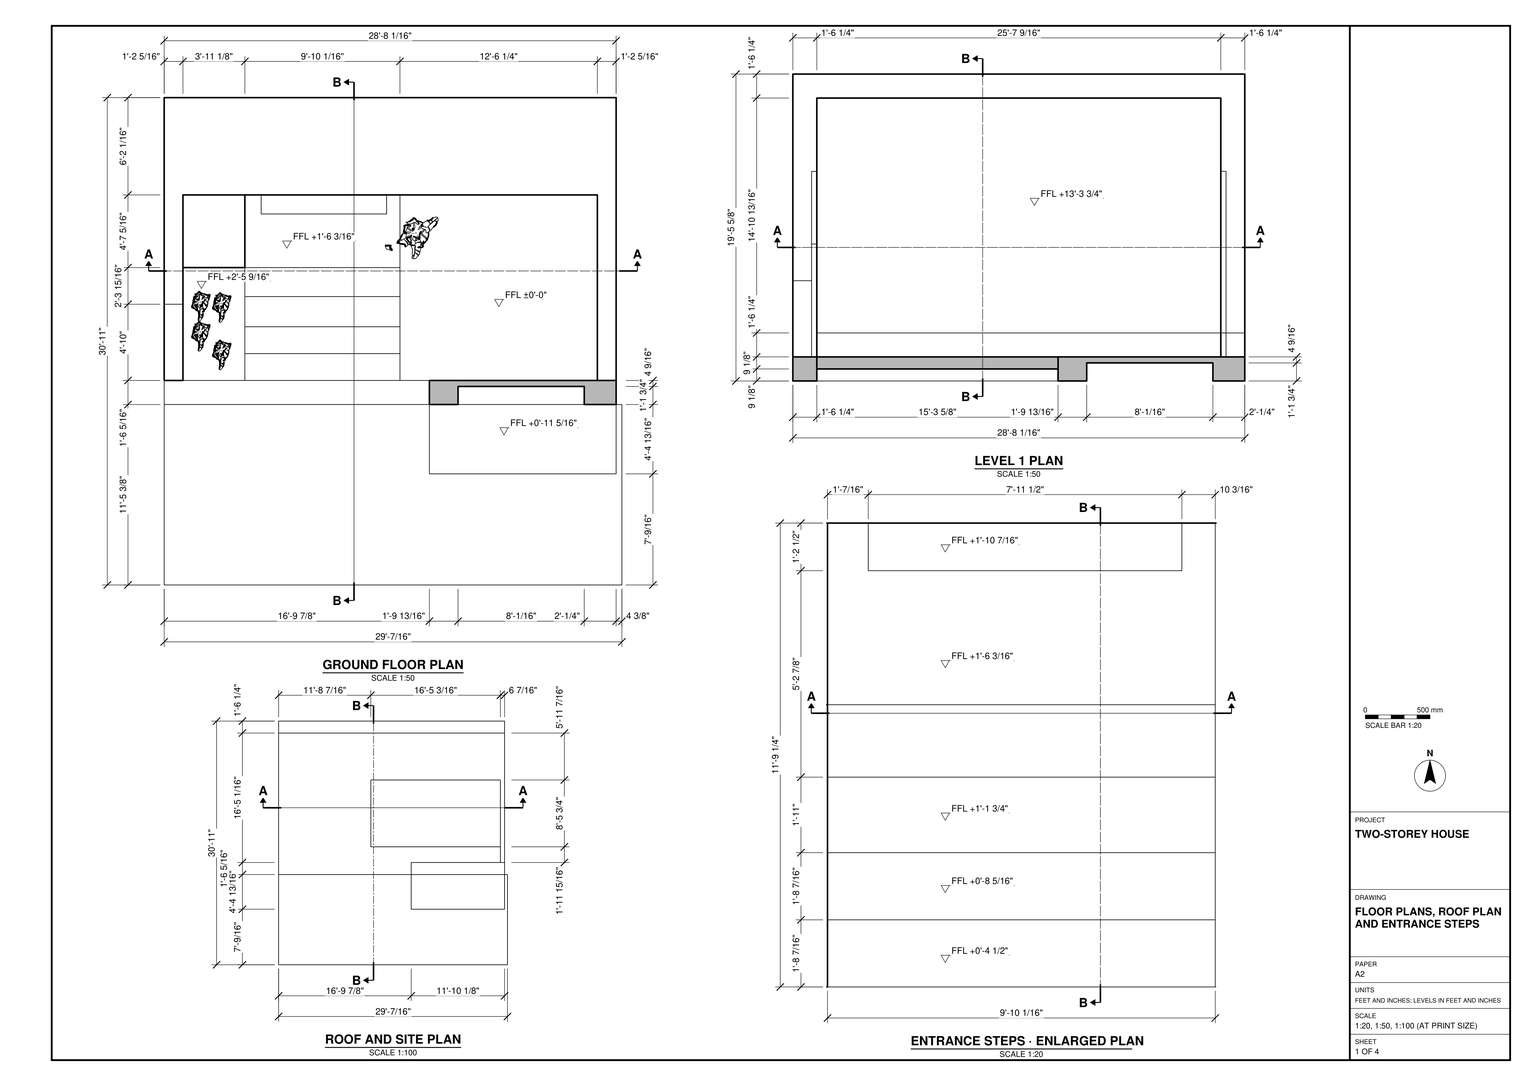
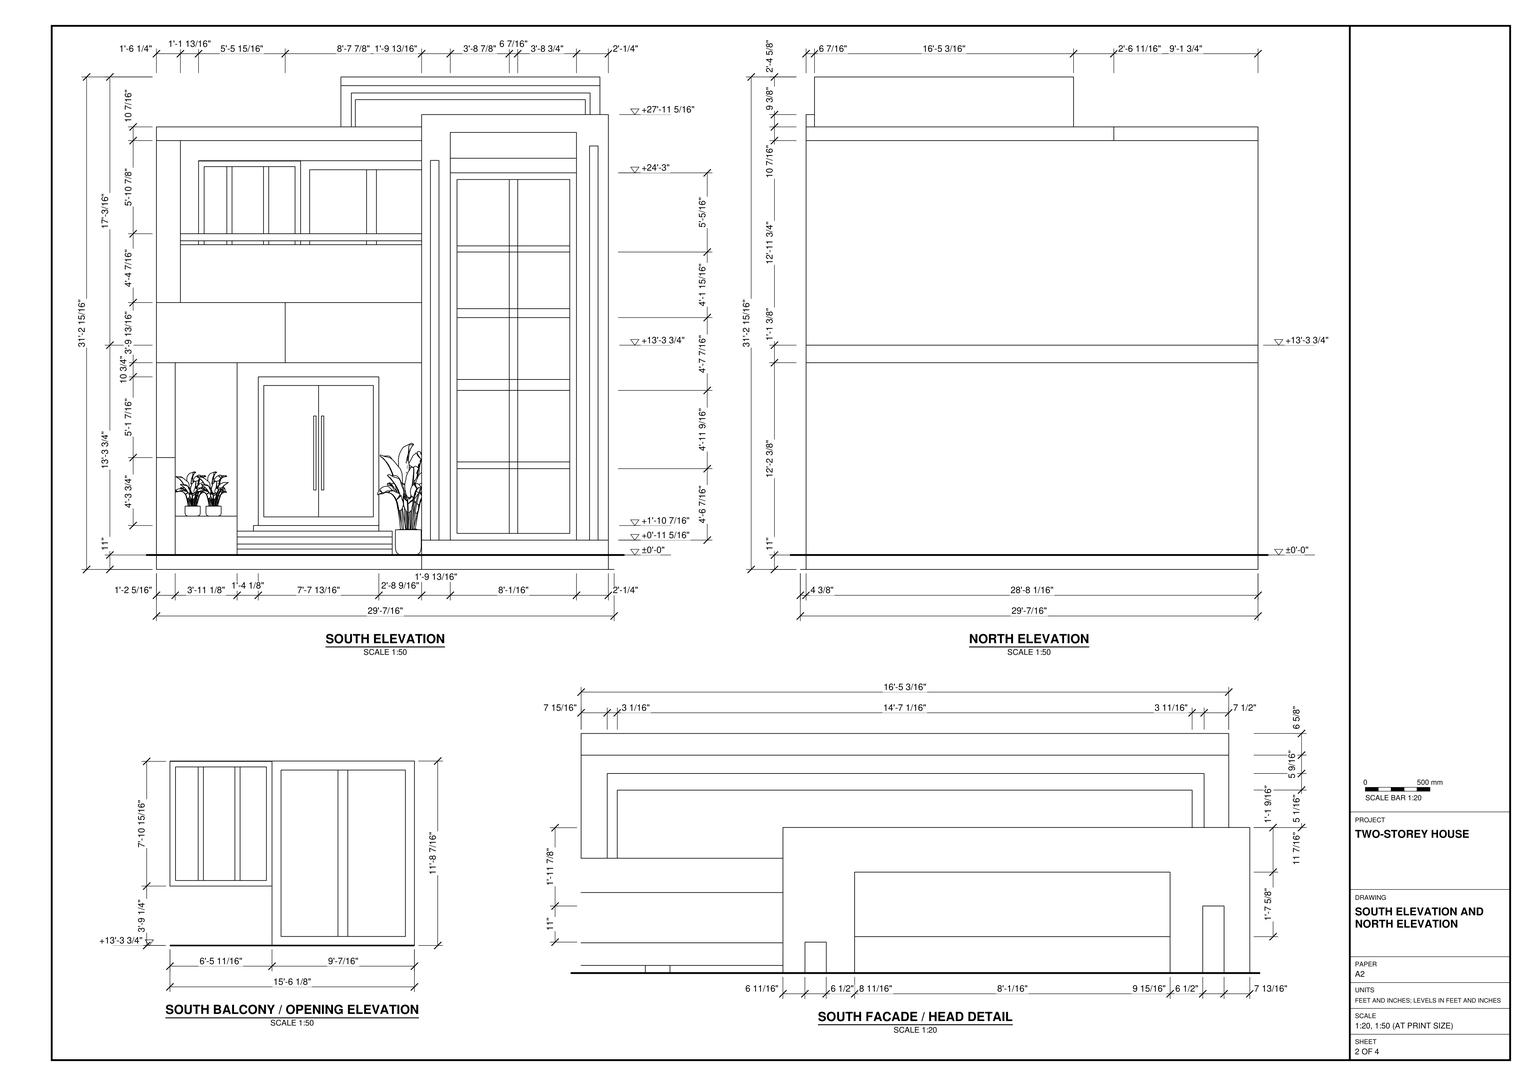
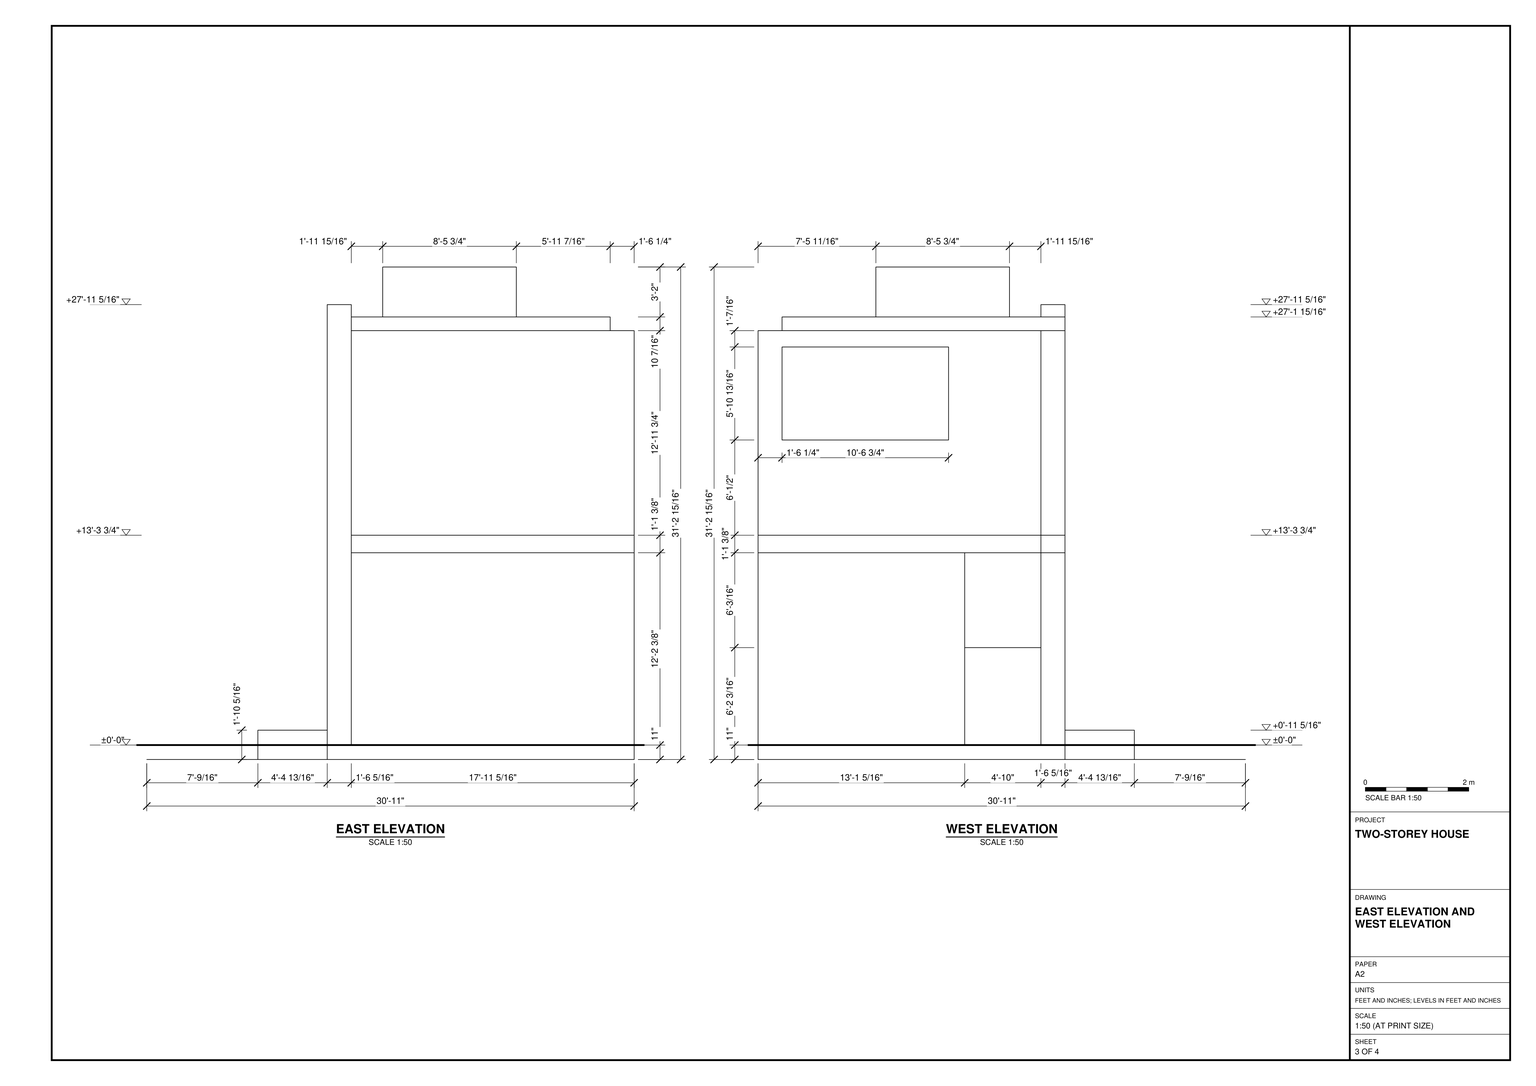
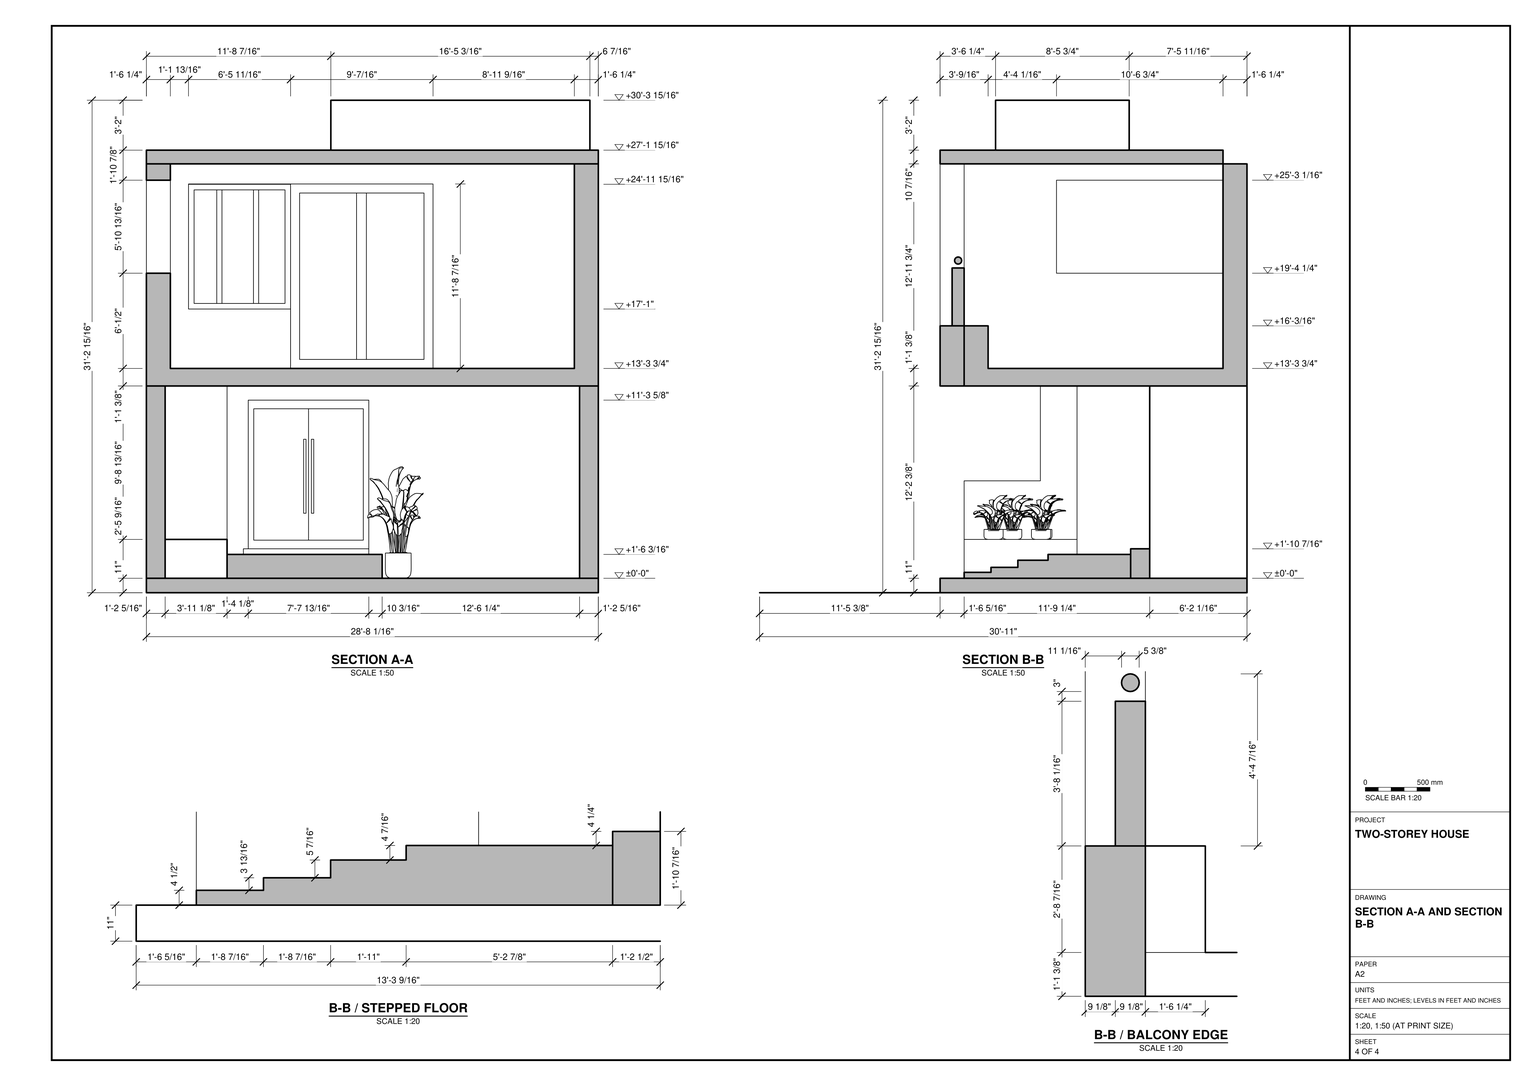
Build the two-storey house in SketchUp from task_files/diagram_01.pdf. Work in feet and inches. Make the overall model 29'-7/16" wide along X, 30'-11" deep along Y and 31'-2 15/16" high along Z. Use ±0'-0" as the ground-floor datum and +13'-3 3/4" as the upper finished floor level.

Set the house on the rectangular site base with the approach on the south side. Use the plans for the wall thicknesses and slab footprints, and the elevations for the slab edges and roof profile. Reproduce the broad entrance steps, deep landing and narrower doorstep beneath the paired entrance doors. Include the raised planting area to the left of the steps and the projecting platform in front of the tall right-hand bay.

Model the upper south balcony with its parapet and the framed openings behind it. Carry the projecting frame of the adjacent tall bay past the upper floor, and divide its inset face as shown in the south elevation. Follow the roof plan and head detail for the raised rectangular roof feature. Any suitable library components may be used for plants and loose decorative items.

Keep walls, slabs, roof elements and each furniture or joinery piece in separate groups or components, and use components for repeated parts. Save one SketchUp model as output_files/two_storey_house_with_a_stepped_entrance_and_balcony.skp.

# SketchUp Ruby script. Lengths in inches.
U = 1.inch
M = Sketchup.active_model
def pt(a) = Geom::Point3d.new(a.map { |v| v * U })
def face(e, loops, mat)
  f = e.add_face(loops[0].map { |a| pt(a) })
  loops[1..].each { |l| e.add_face(l.map { |a| pt(a) }).erase! }
  f.material = f.back_material = mat if mat
  f
end
# faces: each face lists its corners as indices into pts; further lists are holes
def faces(e, pts, list, mat = nil) = list.each { |f| face(e, (f[0].is_a?(Array) ? f : [f]).map { |l| l.map { |i| pts[i] } }, mat) }
# xy, xz, yz: faces in a plane at the given z, y or x. An outline is a flat list of corners, or four numbers for a rectangle; further outlines are holes
def ring(l) = l.size == 4 ? [[l[0], l[1]], [l[2], l[1]], [l[2], l[3]], [l[0], l[3]]] : l.each_slice(2).to_a
def flat(e, list, mat, &to3) = list.each { |f| face(e, (f[0].is_a?(Array) ? f : [f]).map { |l| ring(l).map { |u, v| to3.(u, v) } }, mat) }
def xy(e, z, list, mat = nil) = flat(e, list, mat) { |x, y| [x, y, z] }
def xz(e, y, list, mat = nil) = flat(e, list, mat) { |x, z| [x, y, z] }
def yz(e, x, list, mat = nil) = flat(e, list, mat) { |y, z| [x, y, z] }
def lines(e, pts, list) = list.each { |a, b| e.add_line(pt(pts[a]), pt(pts[b])) }
# prism: a flat outline (further loops are holes) pulled along v
def prism(e, loops, v, mat = nil)
  f = face(e, loops, mat); d = Geom::Vector3d.new(v.map { |x| x * U })
  f.pushpull(f.normal.samedirection?(d) ? d.length : -d.length)
end
def box(e, o, s, mat = nil) = prism(e, [[o, [o[0] + s[0], o[1], o[2]], [o[0] + s[0], o[1] + s[1], o[2]], [o[0], o[1] + s[1], o[2]]]], [0, 0, s[2]], mat)
def at(x, y, z, deg = 0) = Geom::Transformation.translation(pt([x, y, z])) * Geom::Transformation.rotation(ORIGIN, Z_AXIS, deg.degrees)
def axes(o, x, y, z) = Geom::Transformation.new([*x, 0, *y, 0, *z, 0, *pt(o).to_a, 1])
def part(name) = M.definitions.add(name)
# library, detail: a bought-in or finely detailed component or shape, given as its bounding box
def library(name, o, s) = part(name).tap { |d| box(d.entities, o, s) }
def detail(e, o, s) = box(e.add_group.entities, o, s)
def put(e, d, t, mat = nil) = e.add_instance(d, t).tap { |i| i.material = mat if mat }
def group(e, t, mat = nil) = e.add_group.tap { |g| g.transformation = t; g.material = mat if mat }.entities
root = M.entities
M.materials.add("[0012_Bisque]").color = [255, 228, 196]
M.materials.add("[0035_Tan]").color = [210, 180, 140]
M.materials.add("[Asphalt New]").color = [67, 60, 62]
M.materials.add("[Cladding Siding White]").color = [119, 119, 119]
M.materials.add("[Field Rectangle Tile]").color = [196, 189, 179]
M.materials.add("[Field Square Tile]").color = [217, 201, 169]
M.materials.add("[Formica Beige]").color = [211, 187, 149]
M.materials.add("[Formica Laminate Dark]").color = [50, 53, 60]
M.materials.add("[Formica Speckled Grey]").color = [90, 101, 107]
M.materials.add("[Formica Speckled Grey]1").color = [94, 105, 111]
M.materials.add("[Grass Dark Green]").color = [106, 157, 55]
M.materials.add("[Marble Carrara Gold Floor Tile]").color = [225, 223, 217]
M.materials.add("[Polished Concrete Old]").color = [229, 229, 229]
M.materials.add("[Quartz Light Brown]").color = [199, 184, 152]
M.materials.add("[Stone Coursed Rough]").color = [165, 160, 130]
M.materials.add("[Terrazzo Tile Light]").color = [219, 217, 210]
M.materials.add("[Translucent Glass Gray]").color = [128, 128, 128]
M.materials["[Translucent Glass Gray]"].alpha = 0.5
M.materials.add("[Translucent Glass Safety]").color = [204, 235, 244]
M.materials["[Translucent Glass Safety]"].alpha = 0.5
M.materials.add("[Wood Bamboo]").color = [177, 105, 43]
M.materials.add("[Wood Cherry Original]").color = [76, 43, 21]
M.materials.add("[Wood Floor Light]").color = [204, 176, 127]
M.materials.add("[Wood Floor]").color = [58, 39, 23]
M.materials.add("[Wood Veneer 01]").color = [120, 70, 37]
c1 = library("chau cay",[-24.34,-109.24,0],[56.46,62.58,79.69])
xy(root,0,[[201.89,84.57,344.04,137.375],[0,137.375,344.04,371.01]])
xy(root,0,[[0,0,0,137.375,201.89,137.375,201.89,84.57,344.04,84.57,344.04,137.375,348.4375,137.375,348.4375,0]],"[Field Rectangle Tile]")
xy(root,10.98,[[0,155.6875,14.28,213.72],[329.76,155.6875,329.76,296.95,14.28,296.95,14.28,213.72,0,213.72,0,371.01,344.04,371.01,344.04,155.6875],[14.28,155.6875,61.42,241.64],[61.42,155.6875,61.42,296.95,73.83,296.95,73.83,282.45,169.33,282.45,169.33,296.95,179.49,296.95,179.49,155.6875],[14.28,241.64,61.42,296.95],
  [73.83,282.45,169.33,296.95]])
xy(root,10.98,[[0,137.375,201.89,155.6875]],"[Field Rectangle Tile]")
xy(root,10.98,[[179.49,155.6875,329.76,296.95]],"[Field Square Tile]")
xy(root,15.49,[[61.42,155.6875,179.49,176.13]],"[Marble Carrara Gold Floor Tile]")
xy(root,19.31,[[61.42,176.13,179.49,196.58]],"[Marble Carrara Gold Floor Tile]")
xy(root,22.3125,[[223.71,137.375,319.77,151.125]],"[Asphalt New]")
xy(root,22.3125,[[201.89,84.57,344.04,137.375]],"[Grass Dark Green]")
xy(root,24.72,[[61.42,196.58,179.49,219.57]],"[Marble Carrara Gold Floor Tile]")
xy(root,29.14,[[61.42,219.57,179.49,241.64],[61.42,241.64,179.49,241.64,179.49,296.95,169.33,296.95,169.33,282.45,73.83,282.45,73.83,296.95,61.42,296.95]],"[Marble Carrara Gold Floor Tile]")
xy(root,33.42,[[73.83,282.45,169.33,296.95]],"[Marble Carrara Gold Floor Tile]")
xy(root,40.56,[[14.28,155.6875,61.42,241.64]],"[Polished Concrete Old]")
xy(root,85.17,[[0,155.6875,14.28,213.72]],"[0035_Tan]")
xy(root,157.38,[[329.76,155.6875,329.76,296.95,14.28,296.95,14.28,213.72,0,213.72,0,371.01,344.04,371.01,344.04,155.6875],[14.28,241.64,61.42,296.95]])
xy(root,157.38,[[0,137.375,14.28,155.6875],[14.28,137.375,201.89,155.6875],[0,155.6875,14.28,213.72],[14.28,155.6875,14.28,241.64,61.42,241.64,61.42,296.95,329.76,296.95,329.76,155.6875]],"[0012_Bisque]")
xy(root,170.72,[[18.25,173.9375,325.79,352.76]],"[Terrazzo Tile Light]")
xy(root,203.16,[[18.25,146.53,201.89,155.6875],[18.25,155.6875,325.79,173.9375]])
xy(root,203.16,[[18.25,137.375,201.89,146.53]],"[Formica Speckled Grey]1")
xy(root,243.22,[[0,226,18.25,352.76]],"[0035_Tan]")
xy(root,247.22,[[18.25,146.53,201.89,155.6875]],"[Translucent Glass Safety]")
xy(root,301.95,[[223.71,137.375,319.77,151.125]])
xy(root,313.04,[[223.71,137.375,319.77,144.5]],"[Formica Speckled Grey]")
xy(root,314.05,[[0,226,18.25,352.76]],"[0035_Tan]")
xy(root,326.47,[[0,137.375,18.25,155.6875],[0,155.6875,18.25,352.76],[325.79,155.6875,344.04,173.9375],[325.79,173.9375,344.04,352.76]])
xy(root,326.47,[[18.25,137.375,18.25,352.76,325.79,352.76,325.79,155.6875,201.89,155.6875,201.89,137.375]],"[0012_Bisque]")
xy(root,326.47,[[0,352.76,344.04,371.01]],"[0035_Tan]")
xy(root,332.6875,[[223.71,137.375,319.77,144.5]],"[Formica Speckled Grey]")
xy(root,336.91,[[140.43,179.61,337.63,281.33]])
xy(root,336.91,[[0,137.375,201.89,137.375,201.89,155.6875,337.63,155.6875,337.63,179.61,140.43,179.61,140.43,281.33,337.63,281.33,337.63,155.6875,344.04,155.6875,344.04,352.76,0,352.76]],"[0035_Tan]")
xy(root,346.29,[[201.89,137.375,344.04,155.6875]],"[Formica Speckled Grey]1")
xy(root,374.91,[[140.43,179.61,337.63,281.33]],"[Formica Laminate Dark]")
xz(root,84.57,[[201.89,0,344.04,22.3125]],"[Asphalt New]")
xz(root,137.375,[[201.89,0,344.04,22.3125]])
xz(root,137.375,[[0,203.16,18.25,326.47],[0,326.47,201.89,336.91]],"[0035_Tan]")
xz(root,137.375,[[0,157.38,98.03,203.16],[98.03,157.38,201.89,203.16]],"[Cladding Siding White]")
xz(root,137.375,[[0,0,201.89,10.98]],"[Field Rectangle Tile]")
xz(root,137.375,[[223.71,301.95,319.77,313.04]],"[Formica Laminate Dark]")
xz(root,137.375,[[201.89,22.3125,208.59,22.3125,208.59,311.375,215.09,311.375,215.09,22.3125,223.71,22.3125,223.71,332.6875,319.77,332.6875,319.77,22.3125,329.71,22.3125,329.71,322.375,336.21,322.375,336.21,22.3125,344.04,22.3125,344.04,346.29,201.89,346.29]],"[Formica Speckled Grey]")
xz(root,137.375,[[208.59,22.3125,215.09,311.375],[329.71,22.3125,336.21,322.375]],"[Quartz Light Brown]")
xz(root,144.5,[[223.71,313.04,319.77,332.6875]],"[Formica Speckled Grey]")
xz(root,146.53,[[18.25,203.16,201.89,247.22]],"[Translucent Glass Safety]")
xz(root,151.125,[[228.8,27.41,268.61,76.72],[275.02,27.41,314.67,76.72],[228.8,81.86,268.61,136.3],[275.02,81.86,314.67,136.3],[228.8,144.62,268.61,191.74],
  [275.02,144.62,314.67,191.74],[228.8,198.52,268.61,241.65],[275.02,198.52,314.67,241.65],[228.8,246.33,268.61,296.85],[275.02,246.33,314.67,296.85]],"[Translucent Glass Gray]")
xz(root,151.125,[[[223.71,22.3125,319.77,301.95],[228.8,27.41,314.67,296.85]],[268.61,27.41,275.02,76.72],[228.8,76.72,268.61,81.86],[268.61,76.72,275.02,81.86],[275.02,76.72,314.67,81.86],
  [268.61,81.86,275.02,136.3],[228.8,136.3,268.61,144.62],[268.61,136.3,275.02,144.62],[275.02,136.3,314.67,144.62],[268.61,144.62,275.02,191.74],
  [228.8,191.74,268.61,198.52],[268.61,191.74,275.02,198.52],[275.02,191.74,314.67,198.52],[268.61,198.52,275.02,241.65],[228.8,241.65,268.61,246.33],
  [268.61,241.65,275.02,246.33],[275.02,241.65,314.67,246.33],[268.61,246.33,275.02,296.85]],"[Wood Floor]")
xz(root,155.6875,[[329.76,10.98,344.04,157.38],[0,157.38,0,326.47,18.25,326.47,18.25,203.16,201.89,203.16,201.89,157.38],[201.89,157.38,329.76,170.72],[329.76,157.38,344.04,170.72],[201.89,170.72,344.04,203.16],
  [325.79,203.16,344.04,326.47],[201.89,326.47,325.79,336.91],[325.79,326.47,344.04,336.91]])
xz(root,155.6875,[[0,10.98,14.28,85.17]],"[0035_Tan]")
xz(root,155.6875,[[201.89,10.98,329.76,157.38],[201.89,203.16,325.79,326.47],[201.89,336.91,344.04,346.29]],"[Formica Speckled Grey]1")
xz(root,155.6875,[[61.42,10.98,179.49,15.49]],"[Marble Carrara Gold Floor Tile]")
xz(root,155.6875,[[14.28,10.98,61.42,40.56]],"[Polished Concrete Old]")
xz(root,155.6875,[[18.25,203.16,201.89,247.22]],"[Translucent Glass Safety]")
xz(root,173.9375,[[18.25,170.72,325.79,203.16]])
xz(root,176.13,[[61.42,15.49,179.49,19.31]],"[Marble Carrara Gold Floor Tile]")
xz(root,179.61,[[148.38,336.91,151.43,336.91,151.43,357.66,326.49,357.66,326.49,336.91,330.13,336.91,330.13,362.72,148.38,362.72]],"[Formica Beige]")
xz(root,179.61,[[151.43,336.91,326.49,357.66],[140.43,368.3,337.63,374.91]],"[Formica Laminate Dark]")
xz(root,179.61,[[140.43,336.91,148.38,336.91,148.38,362.72,330.13,362.72,330.13,336.91,337.63,336.91,337.63,368.3,140.43,368.3]],"[Formica Speckled Grey]")
xz(root,196.58,[[61.42,19.31,179.49,24.72]],"[Marble Carrara Gold Floor Tile]")
xz(root,213.72,[[0,85.17,14.28,157.38]],"[0035_Tan]")
xz(root,219.57,[[61.42,24.72,179.49,29.14]],"[Marble Carrara Gold Floor Tile]")
xz(root,226,[[0,243.22,18.25,314.05]])
xz(root,241.64,[[14.28,10.98,61.42,40.56]])
xz(root,241.64,[[14.28,40.56,61.42,157.38]],"[Stone Coursed Rough]")
xz(root,281.33,[[140.43,336.91,337.63,374.91]],"[Formica Laminate Dark]")
xz(root,282.45,[[73.83,10.98,169.33,29.14]])
xz(root,282.45,[[73.83,29.14,169.33,33.42]],"[Marble Carrara Gold Floor Tile]")
xz(root,296.95,[[14.28,10.98,61.42,157.38],[61.42,10.98,73.83,29.14],[73.83,10.98,169.33,33.42],[169.33,10.98,179.49,29.14]])
xz(root,296.95,[[179.49,10.98,329.76,10.98,329.76,157.38,61.42,157.38,61.42,29.14,73.83,29.14,73.83,33.42,77.54,33.42,77.54,146.61,169.33,146.61,169.33,29.14,179.49,29.14]],"[0035_Tan]")
xz(root,296.95,[[[81.74,39.99,123.43,140.03],[119.71,60.49,121.51,116.83]],[[123.43,39.99,165.125,140.03],[125.61,60.49,127.41,116.83]]],"[Wood Bamboo]")
xz(root,296.95,[[119.71,60.49,121.51,116.83],[125.61,60.49,127.41,116.83]],"[Wood Floor Light]")
xz(root,296.95,[[[77.54,33.42,169.33,146.61],[81.74,39.99,165.125,140.03]]],"[Wood Veneer 01]")
xz(root,352.76,[[32.07,310.92,109.77,311.16]])
xz(root,352.76,[[18.25,170.72,109.77,170.72,109.77,215.96,32.07,215.96,32.07,311.16,218.21,311.16,218.21,170.72,325.79,170.72,325.79,326.47,18.25,326.47],[0,243.22,18.25,314.05],[0,326.47,109.77,336.91],[109.77,326.47,344.04,336.91]],"[0035_Tan]")
xz(root,352.76,[[116.65,177.6,159.98,304.28]],"[Translucent Glass Gray]")
xz(root,352.76,[[36.3125,220.2,53.58,306.68],[57.54,220.2,81.51,306.68],[85.48,220.2,105.53,306.68]],"[Translucent Glass Safety]")
xz(root,352.76,[[[109.77,170.72,218.21,311.16],[116.65,177.6,211.33,304.28]],[159.98,177.6,167.48,304.28],[[32.07,215.96,109.77,310.92],[36.3125,220.2,105.53,306.68]],[53.58,220.2,57.54,306.68],[81.51,220.2,85.48,306.68]],"[Wood Cherry Original]")
xz(root,352.76,[[167.48,177.6,211.33,304.28]],"[Wood Veneer 01]")
xz(root,371.01,[[0,0,344.04,10.98],[0,10.98,344.04,157.38],[0,157.38,344.04,170.72],[0,170.72,344.04,326.47]],"[0035_Tan]")
yz(root,0,[[137.375,0,371.01,10.98],[155.6875,10.98,213.72,85.17],[213.72,10.98,371.01,157.38],[137.375,157.38,155.6875,170.72],[155.6875,157.38,371.01,170.72],
  [137.375,170.72,155.6875,326.47],[[155.6875,170.72,371.01,326.47],[226,243.22,352.76,314.05]],[137.375,326.47,352.76,336.91]],"[0035_Tan]")
yz(root,14.28,[[155.6875,10.98,213.72,40.56],[213.72,10.98,241.64,40.56],[241.64,10.98,296.95,157.38]])
yz(root,14.28,[[155.6875,40.56,241.64,40.56,241.64,157.38,213.72,157.38,213.72,85.17,155.6875,85.17]],"[0035_Tan]")
yz(root,18.25,[[146.53,203.16,155.6875,247.22]])
yz(root,18.25,[[173.9375,170.72,352.76,170.72,352.76,243.22,226,243.22,226,314.05,352.76,314.05,352.76,326.47,155.6875,326.47,155.6875,203.16,173.9375,203.16],[[137.375,203.16,146.53,203.16,146.53,247.22,155.6875,247.22,155.6875,326.47,137.375,326.47],[151.11,250.19,150.41,250.28,149.76,250.55,149.21,250.98,148.78,251.54,148.51,252.18,148.42,252.88,148.51,253.58,148.78,254.22,149.21,254.78,149.76,255.21,150.41,255.48,151.11,255.57,151.8,255.48,152.45,255.21,153.01,254.78,153.4375,254.22,153.7,253.58,153.8,252.88,153.7,252.18,153.4375,251.54,153.01,250.98,152.45,250.55,151.8,250.28]]],"[0035_Tan]")
yz(root,61.42,[[155.6875,10.98,241.64,10.98,241.64,29.14,219.57,29.14,219.57,24.72,196.58,24.72,196.58,19.31,176.13,19.31,176.13,15.49,155.6875,15.49],[241.64,10.98,296.95,29.14]])
yz(root,61.42,[[241.64,29.14,296.95,157.38]],"[0035_Tan]")
yz(root,61.42,[[155.6875,15.49,176.13,15.49,176.13,19.31,196.58,19.31,196.58,24.72,219.57,24.72,219.57,29.14,241.64,29.14,241.64,40.56,155.6875,40.56]],"[Polished Concrete Old]")
yz(root,73.83,[[282.45,10.98,296.95,29.14]])
yz(root,73.83,[[282.45,29.14,296.95,33.42]],"[Marble Carrara Gold Floor Tile]")
yz(root,140.43,[[179.61,336.91,281.33,374.91]],"[Formica Laminate Dark]")
yz(root,169.33,[[282.45,10.98,296.95,29.14]])
yz(root,169.33,[[282.45,29.14,296.95,33.42]],"[Marble Carrara Gold Floor Tile]")
yz(root,179.49,[[155.6875,10.98,296.95,10.98,296.95,29.14,219.57,29.14,219.57,24.72,196.58,24.72,196.58,19.31,176.13,19.31,176.13,15.49,155.6875,15.49]])
yz(root,201.89,[[137.375,157.38,155.6875,170.72],[137.375,170.72,155.6875,203.16],[146.53,203.16,155.6875,247.22],[151.11,250.19,151.8,250.28,152.45,250.55,153.01,250.98,153.4375,251.54,153.7,252.18,153.8,252.88,153.7,253.58,153.4375,254.22,153.01,254.78,152.45,255.21,151.8,255.48,151.11,255.57,150.41,255.48,149.76,255.21,149.21,254.78,148.78,254.22,148.51,253.58,148.42,252.88,148.51,252.18,148.78,251.54,149.21,250.98,149.76,250.55,150.41,250.28],[137.375,326.47,155.6875,336.91]])
yz(root,201.89,[[84.57,0,137.375,22.3125]],"[Asphalt New]")
yz(root,201.89,[[137.375,10.98,155.6875,157.38],[[137.375,203.16,137.375,326.47,155.6875,326.47,155.6875,247.22,146.53,247.22,146.53,203.16],[151.11,250.19,151.8,250.28,152.45,250.55,153.01,250.98,153.4375,251.54,153.7,252.18,153.8,252.88,153.7,253.58,153.4375,254.22,153.01,254.78,152.45,255.21,151.8,255.48,151.11,255.57,150.41,255.48,149.76,255.21,149.21,254.78,148.78,254.22,148.51,253.58,148.42,252.88,148.51,252.18,148.78,251.54,149.21,250.98,149.76,250.55,150.41,250.28]],[137.375,336.91,155.6875,346.29]],"[Formica Speckled Grey]1")
yz(root,223.71,[[137.375,22.3125,151.125,301.95]],"[Formica Laminate Dark]")
yz(root,223.71,[[137.375,313.04,144.5,332.6875]],"[Formica Speckled Grey]")
yz(root,319.77,[[137.375,22.3125,151.125,301.95]],"[Formica Laminate Dark]")
yz(root,319.77,[[137.375,313.04,144.5,332.6875]],"[Formica Speckled Grey]")
yz(root,325.79,[[173.9375,170.72,173.9375,203.16,155.6875,203.16,155.6875,326.47,352.76,326.47,352.76,170.72]],"[0035_Tan]")
yz(root,329.76,[[155.6875,10.98,296.95,157.38]],"[0035_Tan]")
yz(root,337.63,[[179.61,336.91,281.33,374.91]],"[Formica Laminate Dark]")
yz(root,344.04,[[155.6875,10.98,371.01,157.38],[155.6875,157.38,371.01,170.72],[155.6875,170.72,371.01,326.47],[155.6875,326.47,352.76,336.91]],"[0035_Tan]")
yz(root,344.04,[[84.57,0,137.375,22.3125]],"[Asphalt New]")
yz(root,344.04,[[137.375,0,371.01,0,371.01,10.98,155.6875,10.98,155.6875,346.29,137.375,346.29]],"[Formica Speckled Grey]1")
p = [[201.89,151.11,250.19],[201.89,150.41,250.28],[18.25,150.41,250.28],[18.25,151.11,250.19],[201.89,151.8,250.28],[18.25,151.8,250.28],
  [201.89,149.76,250.55],[18.25,149.76,250.55],[201.89,152.45,250.55],[18.25,152.45,250.55],[201.89,149.21,250.98],[18.25,149.21,250.98],
  [201.89,153.01,250.98],[18.25,153.01,250.98],[201.89,148.78,251.54],[18.25,148.78,251.54],[201.89,153.4375,251.54],[18.25,153.4375,251.54],
  [201.89,148.51,252.18],[18.25,148.51,252.18],[201.89,153.7,252.18],[18.25,153.7,252.18],[201.89,148.42,252.88],[18.25,148.42,252.88],
  [201.89,153.8,252.88],[18.25,153.8,252.88],[201.89,148.51,253.58],[18.25,148.51,253.58],[201.89,153.7,253.58],[18.25,153.7,253.58],
  [201.89,148.78,254.22],[18.25,148.78,254.22],[201.89,153.4375,254.22],[18.25,153.4375,254.22],[201.89,149.21,254.78],[18.25,149.21,254.78],
  [201.89,153.01,254.78],[18.25,153.01,254.78],[201.89,149.76,255.21],[18.25,149.76,255.21],[201.89,152.45,255.21],[18.25,152.45,255.21],
  [201.89,150.41,255.48],[18.25,150.41,255.48],[201.89,151.8,255.48],[18.25,151.8,255.48],[201.89,151.11,255.57],[18.25,151.11,255.57],
  [18.25,173.9375,170.72],[18.25,155.6875,170.72],[325.79,173.9375,170.72],[344.04,173.9375,170.72],[325.79,173.9375,203.16],[344.04,173.9375,203.16]]
faces(root,p,[[0,1,2,3],[4,0,3,5],[1,6,7,2],[8,4,5,9],[6,10,11,7],[12,8,9,13],[10,14,15,11],[16,12,13,17],
  [14,18,19,15],[20,16,17,21],[18,22,23,19],[24,20,21,25],[22,26,27,23],[28,24,25,29],[26,30,31,27],[32,28,29,33],
  [30,34,35,31],[36,32,33,37],[34,38,39,35],[40,36,37,41],[38,42,43,39],[44,40,41,45],[42,46,47,43],[46,44,45,47]],"[Formica Laminate Dark]")
lines(root,p,[[48,49],[50,51],[52,53]])
put(root,c1,axes([189.97,346.53,10.98],[1,0,0],[0,1,0],[0,0,1.15]))
put(root,c1,axes([26.53,273.66,40.57],[0.59,0,0],[0,0.74,0],[0,0,0.45643]))
put(root,c1,axes([26.53,250.72,40.57],[0.59,0,0],[0,0.74,0],[0,0,0.45643]))
put(root,c1,axes([42.47,272.64,40.57],[0.59,0,0],[0,0.74,0],[0,0,0.45643]))
put(root,c1,axes([42.47,236.52,40.57],[0.59,0,0],[0,0.74,0],[0,0,0.45643]))
